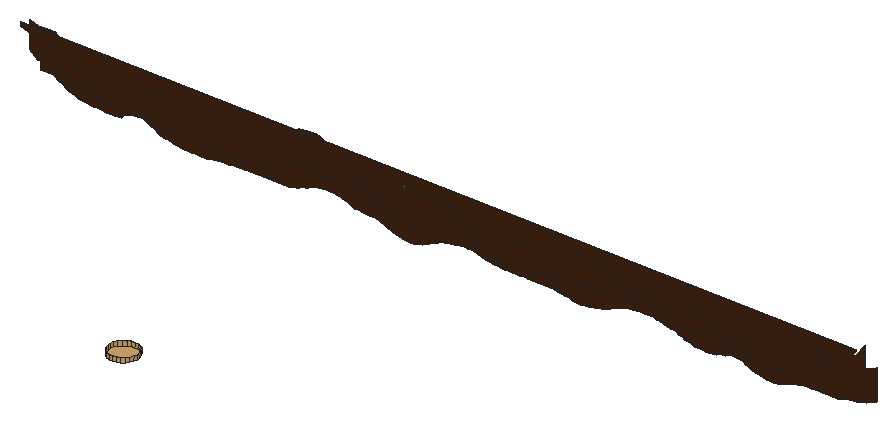
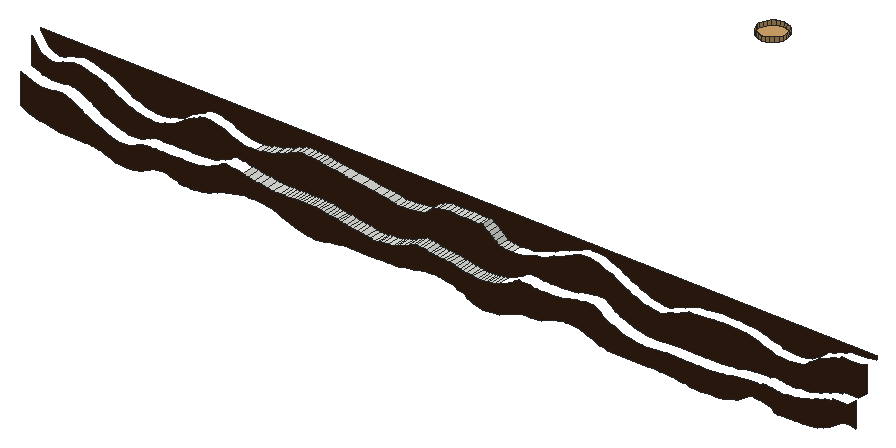
# SketchUp Ruby script. Lengths in inches.
U = 1.inch
M = Sketchup.active_model
def pt(a) = Geom::Point3d.new(a.map { |v| v * U })
def face(e, loops, mat)
  f = e.add_face(loops[0].map { |a| pt(a) })
  loops[1..].each { |l| e.add_face(l.map { |a| pt(a) }).erase! }
  f.material = f.back_material = mat if mat
  f
end
# faces: each face lists its corners as indices into pts; further lists are holes
def faces(e, pts, list, mat = nil) = list.each { |f| face(e, (f[0].is_a?(Array) ? f : [f]).map { |l| l.map { |i| pts[i] } }, mat) }
# xy, xz, yz: faces in a plane at the given z, y or x. An outline is a flat list of corners, or four numbers for a rectangle; further outlines are holes
def ring(l) = l.size == 4 ? [[l[0], l[1]], [l[2], l[1]], [l[2], l[3]], [l[0], l[3]]] : l.each_slice(2).to_a
def flat(e, list, mat, &to3) = list.each { |f| face(e, (f[0].is_a?(Array) ? f : [f]).map { |l| ring(l).map { |u, v| to3.(u, v) } }, mat) }
def xy(e, z, list, mat = nil) = flat(e, list, mat) { |x, y| [x, y, z] }
def xz(e, y, list, mat = nil) = flat(e, list, mat) { |x, z| [x, y, z] }
def yz(e, x, list, mat = nil) = flat(e, list, mat) { |y, z| [x, y, z] }
def lines(e, pts, list) = list.each { |a, b| e.add_line(pt(pts[a]), pt(pts[b])) }
# prism: a flat outline (further loops are holes) pulled along v
def prism(e, loops, v, mat = nil)
  f = face(e, loops, mat); d = Geom::Vector3d.new(v.map { |x| x * U })
  f.pushpull(f.normal.samedirection?(d) ? d.length : -d.length)
end
def box(e, o, s, mat = nil) = prism(e, [[o, [o[0] + s[0], o[1], o[2]], [o[0] + s[0], o[1] + s[1], o[2]], [o[0], o[1] + s[1], o[2]]]], [0, 0, s[2]], mat)
def at(x, y, z, deg = 0) = Geom::Transformation.translation(pt([x, y, z])) * Geom::Transformation.rotation(ORIGIN, Z_AXIS, deg.degrees)
def axes(o, x, y, z) = Geom::Transformation.new([*x, 0, *y, 0, *z, 0, *pt(o).to_a, 1])
def part(name) = M.definitions.add(name)
# library, detail: a bought-in or finely detailed component or shape, given as its bounding box
def library(name, o, s) = part(name).tap { |d| box(d.entities, o, s) }
def detail(e, o, s) = box(e.add_group.entities, o, s)
def put(e, d, t, mat = nil) = e.add_instance(d, t).tap { |i| i.material = mat if mat }
def group(e, t, mat = nil) = e.add_group.tap { |g| g.transformation = t; g.material = mat if mat }.entities
root = M.entities
M.materials.add("[Field Square Tile]").color = [211, 167, 108]
M.materials.add("[Wood Veneer 01]").color = [66, 38, 20]
xy(root,243.05,[[2994.54,2398.8,2995.22,2401.37]])
xy(root,243.07,[[2992.6875,2398.8,2993.27,2401.37]])
xy(root,243.09,[[2989.375,2398.8,2989.9,2401.37],[2989.9,2398.8,2990.42,2401.37],[2990.42,2398.8,2991.08,2401.37],[2991.08,2398.8,2991.53,2401.37]])
xy(root,249.21,[[2962.17,2396.68,2963.06,2398.8]])
xy(root,249.22,[[2963.78,2396.68,2964.6875,2398.8]])
xy(root,249.23,[[2965.33,2396.68,2966.23,2398.8]])
xy(root,250.6875,[[2960.72,2328.39,2960.06,2328.48,2959.44,2328.74,2958.91,2329.14,2958.5,2329.68,2958.25,2330.29,2958.16,2330.96,2958.25,2331.62,2958.5,2332.24,2958.91,2332.77,2959.44,2333.18,2960.06,2333.43,2960.72,2333.52,2961.38,2333.43,2962,2333.18,2962.53,2332.77,2962.94,2332.24,2963.2,2331.62,2963.28,2330.96,2963.2,2330.29,2962.94,2329.68,2962.53,2329.14,2962,2328.74,2961.38,2328.48]],"[Field Square Tile]")
xz(root,2396.68,[[3020.59,244.87,3021.5,245.01,3022.4375,245.12,3023.2,245.25,3023.96,245.41,3024.59,245.78,3025.39,245.88,3026.1,246.16,3026.7,246.57,3027.49,246.9,3028.09,247.35,3028.76,247.62,3029.35,248.06,3030.11,248.32,3031.22,248.66,3032,248.79,3032.86,249.19,3033.53,249.32,3034.46,249.41,3035.31,249.48,3036.06,249.21,3036.7,248.96,3037.4,248.9,3038.2,248.42,3038.91,248.3,3039.62,248.22,3040.4375,248.56,3041.37,249.02,3043.1,251.16,3043.1,251.5,2889.09,251.5,2889.09,250.88,2890.68,250.53,2892.3,250.54,2893.76,250.55,2894.29,250.15,2894.9,249.97,2895.7,249.8,2896.37,249.41,2897.04,249.2,2897.81,249.01,2898.3,248.51,2898.93,248.07,2899.58,247.72,2900.22,247.25,2900.77,246.88,2901.49,246.73,2902.15,246.62,2902.89,246.54,2903.67,246.51,2904.45,246.58,2905.25,246.59,2906.05,246.69,2906.76,247.03,2907.45,247.2,2908.42,247.39,2909.05,247.78,2909.83,247.89,2910.83,248.18,2911.47,248.29,2912.36,248.35,2913.09,248.4,2914.08,248.4375,2914.74,248.46,2915.63,248.47,2916.37,248.48,2917.26,248.49,2917.99,248.39,2919.39,248.28,2920.42,248.15,2921.24,248.11,2922.04,248.08,2922.88,247.66,2923.51,247.46,2924.19,247.08,2924.875,246.94,2925.73,246.66,2926.34,246.35,2927.11,246.05,2928.01,246.13,2928.72,246.29,2929.52,246.41,2930.43,246.55,2931.16,246.92,2931.77,247.12,2932.45,247.31,2933.02,247.71,2933.95,248.03,2934.66,248.46,2935.44,248.82,2936.16,249.37,2936.95,249.5625,2937.85,249.9,2938.77,250.35,2939.43,250.49,2940.24,250.6,2941.26,250.58,2941.9,250.61,2942.52,250.32,2943.21,250.0625,2943.87,249.68,2944.63,249.46,2945.52,248.95,2946.74,248.69,2947.65,248.26,2948.25,247.9,2949.38,247.66,2949.96,247.53,2950.64,247.25,2951.45,246.95,2952.14,246.75,2952.93,246.66,2953.64,246.59,2954.53,246.55,2955.46,246.63,2956.2,246.74,2956.93,246.87,2957.54,247.42,2958.21,247.96,2958.78,248.44,2959.52,248.85,2959.99,249.34,2960.72,249.125,2961.49,249.17,2962.17,249.21,2963.06,249.21,2963.78,249.22,2964.6875,249.22,2965.33,249.23,2966.23,249.23,2966.97,249.24,2967.77,249.14,2968.4,248.82,2969.19,248.54,2969.89,248.04,2970.58,247.48,2971.47,247.29,2972.29,247.15,2973.02,247.05,2973.74,247,2974.65,246.96,2975.375,246.94,2976.29,247.04,2977.35,247.36,2978.53,247.43,2980.18,247.6,2982.16,247.98,2984.36,248.1875,2985.97,248.49,2987.22,248.62,2988.16,248.69,2988.84,248.75,2989.5,249.09,2990.2,249.18,2990.98,249.13,2991.68,249.17,2992.38,249.18,2993.28,249.29,2994.01,249.21,2994.62,248.8,2995.3125,248.73,2996.09,248.26,2996.79,248.02,2997.59,247.8125,2998.3,247.4,2999.21,247.27,2999.95,247.18,3000.875,246.91,3001.74,246.84,3002.69,246.79,3003.47,246.75,3004.22,246.83,3005.26,247.25,3006.13,247.55,3006.8,247.66,3007.43,248.16,3008.22,248.41,3008.92,248.52,3009.62,248.72,3010.32,248.8,3011.21,248.85,3012.04,248.6875,3012.58,248.26,3013.27,248.06,3014.16,247.55,3014.87,247.19,3015.68,246.63,3016.3125,246.13,3016.9,245.83,3017.58,245.67,3018.45,245.46,3019.16,245.0625,3019.875,244.95]],"[Wood Veneer 01]")
xz(root,2398.8,[[3024.59,241.09,3025.16,241.14,3025.8,241.35,3026.39,241.46,3027.33,241.85,3028.33,242.23,3028.89,242.42,3029.61,242.61,3030.125,242.91,3030.5,243.14,3031.04,243.52,3031.52,243.71,3031.85,244.02,3032.29,244.21,3032.88,244.57,3033.35,244.76,3033.97,245.125,3034.47,245.32,3034.95,245.41,3035.5,245.48,3035.99,245.59,3036.52,245.55,3037.13,245.35,3037.62,245.31,3038.17,245.27,3038.73,245.24,3039.29,245.22,3039.85,245.34,3040.48,245.42,3041.0625,245.52,3041.44,245.76,3041.91,245.9,3043.1,246.43,3043.1,251.16,3041.37,249.02,3040.4375,248.56,3039.62,248.22,3038.91,248.3,3038.2,248.42,3037.4,248.9,3036.7,248.96,3036.06,249.21,3035.31,249.48,3034.46,249.41,3033.53,249.32,3032.86,249.19,3032,248.79,3031.22,248.66,3030.11,248.32,3029.35,248.06,3028.76,247.62,3028.09,247.35,3027.49,246.9,3026.7,246.57,3026.1,246.16,3025.39,245.88,3024.59,245.78,3023.96,245.41,3023.2,245.25,3022.4375,245.12,3021.5,245.01,3020.59,244.87,3019.875,244.95,3019.16,245.0625,3018.45,245.46,3017.58,245.67,3016.9,245.83,3016.3125,246.13,3015.68,246.63,3014.87,247.19,3014.16,247.55,3013.27,248.06,3012.58,248.26,3012.04,248.6875,3011.21,248.85,3010.32,248.8,3009.62,248.72,3008.92,248.52,3008.22,248.41,3007.43,248.16,3006.8,247.66,3006.13,247.55,3005.26,247.25,3004.22,246.83,3003.47,246.75,3002.69,246.79,3001.74,246.84,3000.875,246.91,2999.95,247.18,2999.21,247.27,2998.3,247.4,2997.59,247.8125,2996.79,248.02,2996.09,248.26,2995.3125,248.73,2994.62,248.8,2994.01,249.21,2993.28,249.29,2992.38,249.18,2991.68,249.17,2990.98,249.13,2990.2,249.18,2989.5,249.09,2988.84,248.75,2988.16,248.69,2987.22,248.62,2985.97,248.49,2984.36,248.1875,2982.16,247.98,2980.18,247.6,2978.53,247.43,2977.35,247.36,2976.29,247.04,2975.375,246.94,2974.65,246.96,2973.74,247,2973.02,247.05,2972.29,247.15,2971.47,247.29,2970.58,247.48,2969.89,248.04,2969.19,248.54,2968.4,248.82,2967.77,249.14,2966.97,249.24,2966.23,249.23,2965.33,249.23,2964.6875,249.22,2963.78,249.22,2963.06,249.21,2962.17,249.21,2961.49,249.17,2960.72,249.125,2959.99,249.34,2959.52,248.85,2958.78,248.44,2958.21,247.96,2957.54,247.42,2956.93,246.87,2956.2,246.74,2955.46,246.63,2954.53,246.55,2953.64,246.59,2952.93,246.66,2952.14,246.75,2951.45,246.95,2950.64,247.25,2949.96,247.53,2949.38,247.66,2948.25,247.9,2947.65,248.26,2946.74,248.69,2945.52,248.95,2944.63,249.46,2943.87,249.68,2943.21,250.0625,2942.52,250.32,2941.9,250.61,2941.26,250.58,2940.24,250.6,2939.43,250.49,2938.77,250.35,2937.85,249.9,2936.95,249.5625,2936.16,249.37,2935.44,248.82,2934.66,248.46,2933.95,248.03,2933.02,247.71,2932.45,247.31,2931.77,247.12,2931.16,246.92,2930.43,246.55,2929.52,246.41,2928.72,246.29,2928.01,246.13,2927.11,246.05,2926.34,246.35,2925.73,246.66,2924.875,246.94,2924.19,247.08,2923.51,247.46,2922.88,247.66,2922.04,248.08,2921.24,248.11,2920.42,248.15,2919.39,248.28,2917.99,248.39,2917.26,248.49,2916.37,248.48,2915.63,248.47,2914.74,248.46,2914.08,248.4375,2913.09,248.4,2912.36,248.35,2911.47,248.29,2910.83,248.18,2909.83,247.89,2909.05,247.78,2908.42,247.39,2907.45,247.2,2906.76,247.03,2906.05,246.69,2905.25,246.59,2904.45,246.58,2903.67,246.51,2902.89,246.54,2902.15,246.62,2901.49,246.73,2900.77,246.88,2900.22,247.25,2899.58,247.72,2898.93,248.07,2898.3,248.51,2897.81,249.01,2897.04,249.2,2896.37,249.41,2895.7,249.8,2894.9,249.97,2894.29,250.15,2893.76,250.55,2892.3,250.54,2890.68,250.53,2889.09,250.88,2889.09,246.2,2890.66,244.96,2892.05,244.9375,2893.3,244.92,2893.52,244.61,2894.08,244.54,2894.84,244.41,2895.51,244.11,2896.03,243.95,2896.69,243.79,2897.21,243.48,2897.85,243.3,2898.4375,243.14,2898.92,243.06,2899.64,242.85,2900.22,242.78,2901.03,242.73,2901.57,242.68,2902.24,242.51,2902.76,242.46,2903.3,242.58,2903.93,242.57,2904.56,242.81,2905.13,242.86,2905.69,242.89,2906.33,242.92,2906.76,242.625,2907.37,242.65,2907.92,242.62,2908.55,242.58,2909.11,242.57,2909.75,242.48,2910.41,242.38,2911.07,242.34,2911.74,242.24,2912.91,241.96,2913.68,241.89,2914.5,241.83,2915.1,241.78,2915.87,241.75,2916.32,241.74,2916.87,241.72,2918.13,241.7,2918.86,241.69,2919.53,241.68,2920.12,241.68,2920.61,241.67,2921.3125,241.74,2921.88,241.75,2923.88,241.75,2924.37,241.67,2924.9,241.66,2925.51,241.57,2926.05,241.53,2926.67,241.51,2927.22,241.49,2927.92,241.48,2928.58,241.47,2929.15,241.46,2929.86,241.6,2930.59,241.85,2931.26,241.91,2932.16,242.1,2932.93,242.46,2933.63,242.78,2934.4,242.97,2934.93,243.23,2935.33,243.48,2935.85,243.72,2936.1875,244.12,2936.66,244.39,2937.14,244.73,2937.625,244.87,2938.21,244.95,2938.89,245.01,2939.54,244.81,2940.11,244.7,2940.59,244.67,2941.2,244.55,2941.74,244.51,2942.2,244.25,2942.95,244.11,2943.51,244.04,2944.13,243.99,2944.85,243.95,2945.35,243.93,2946.04,243.91,2946.61,243.89,2947.31,243.88,2947.96,243.94,2948.6,243.95,2949.16,244.1,2949.79,244.13,2950.27,244.15,2950.79,244.17,2951.31,244.18,2951.91,243.8,2952.45,243.43,2953.06,243.09,2953.45,242.875,2953.95,242.68,2954.54,242.51,2955.05,242.21,2955.65,242.11,2956.33,241.96,2956.89,241.89,2957.35,241.85,2957.87,241.8125,2958.38,241.79,2958.96,241.78,2959.63,241.91,2960.1,241.93,2960.77,242.09,2961.54,242.2,2962.04,242.24,2962.65,242.42,2963.2,242.47,2963.95,242.71,2964.59,242.78,2965.07,242.82,2965.76,242.85,2966.46,242.87,2967.01,243.02,2967.63,243.05,2968.18,243.29,2968.86,243.35,2969.41,243.39,2970.01,243.42,2970.78,243.14,2971.35,242.9375,2971.9,242.65,2972.52,242.39,2973.28,242.14,2973.92,241.89,2974.41,241.78,2975.46,241.63,2976.23,241.56,2976.83,241.51,2977.28,241.48,2977.8,241.46,2978.67,241.51,2979.39,241.59,2980.33,241.82,2981.11,241.87,2981.875,241.98,2982.49,242.02,2983.14,242.19,2983.84,242.38,2984.33,242.4375,2984.85,242.48,2985.51,242.58,2986.04,242.61,2986.625,242.77,2987.08,242.95,2987.64,243.01,2988.15,243.05,2988.72,243.08,2989.375,243.09,2991.53,243.09,2992.1,243.08,2992.6875,243.07,2993.27,243.07,2993.93,243.0625,2994.54,243.05,2995.22,243.05,2996.49,243.1,2997.66,243.17,2998.8,243.4,3000.0625,243.52,3001.19,243.71,3002.09,243.99,3002.79,244.08,3003.49,244.21,3004.07,244.27,3004.61,244.3,3005.28,244.39,3005.875,244.19,3006.25,243.88,3006.73,243.59,3007.28,243.33,3007.83,243.22,3008.32,242.92,3008.8,242.75,3009.36,242.6,3009.92,242.52,3010.48,242.47,3011.0625,242.43,3011.64,242.4,3012.22,242.39,3012.8,242.37,3013.38,242.36,3013.97,242.35,3015.13,242.33,3015.71,242.33,3016.43,242.32,3016.9,242.3125,3017.54,242.3,3018.21,242.3,3018.66,242.29,3019.3,242.28,3019.8125,242.28,3020.44,242.2,3021.02,241.97,3021.59,241.84,3022.1,241.57,3022.52,241.33,3022.99,241.24,3023.52,241.17,3023.99,241.12]],"[Wood Veneer 01]")
xz(root,2401.37,[[2957.95,236.98,2958.63,237.22,2959.48,237.43,2960.1,237.74,2960.8,238.02,2961.24,238.375,2961.8,238.51,2962.4375,238.76,2963.08,239.12,2963.66,239.22,2964.66,239.31,2965.47,239.54,2965.96,239.6,2966.58,239.65,2967.17,239.69,2967.73,239.7,2968.46,239.72,2969.07,239.56,2969.74,239.44,2970.59,239.16,2971.14,239.07,2971.91,238.93,2972.79,238.78,2973.27,238.73,2973.94,238.6875,2974.63,238.66,2975.3,238.65,2976.08,238.64,2976.7,238.63,2977.39,238.625,2978.25,238.625,2978.81,238.62,2983.7,238.62,2984.39,238.45,2985.15,238.25,2985.77,238.19,2986.54,238.15,2987.17,237.86,2987.94,237.79,2988.65,237.74,2989.52,237.87,2990.17,237.88,2991.29,238.14,2992.51,238.46,2993.26,238.72,2994.14,239.08,2994.93,239.375,2995.67,239.75,2996.32,239.97,2996.94,240.17,2997.62,240.27,2998.3,240.33,2998.99,240.37,2999.68,240.4,3000.375,240.41,3000.9,240.42,3001.48,240.43,3002.05,240.43,3002.7,240.27,3003.28,240.23,3003.93,239.96,3004.6875,239.8,3005.3,239.65,3006.0625,239.5,3006.6875,239.18,3007.37,239.01,3007.89,238.67,3008.46,238.56,3009.12,238.48,3009.6875,238.26,3010.26,238.19,3011.08,238.15,3011.61,238.11,3012.28,238.18,3012.96,238.18,3013.64,238.27,3014.16,238.55,3014.82,238.61,3015.41,238.66,3015.98,239.04,3016.72,239.125,3017.4,239.02,3018.09,238.96,3018.61,238.86,3019.11,238.57,3019.66,238.33,3020.37,238,3021.2,237.71,3021.74,237.59,3022.34,237.51,3022.93,237.45,3023.5,237.42,3024.23,237.4,3024.91,237.47,3025.51,237.5625,3026.2,237.84,3026.88,238.08,3027.57,238.33,3028.1,238.51,3028.67,238.6,3029.33,238.74,3029.91,238.8,3030.48,238.83,3031.22,238.86,3031.98,238.875,3032.52,238.88,3033.2,238.89,3033.88,238.89,3034.64,238.9,3036.03,238.9,3036.66,239.15,3037.43,239.28,3038.23,239.42,3038.95,239.49,3039.5,239.53,3040.1875,239.81,3040.71,239.96,3041.27,240.1,3043.1,240.89,3043.1,246.43,3041.91,245.9,3041.44,245.76,3041.0625,245.52,3040.48,245.42,3039.85,245.34,3039.29,245.22,3038.73,245.24,3038.17,245.27,3037.62,245.31,3037.13,245.35,3036.52,245.55,3035.99,245.59,3035.5,245.48,3034.95,245.41,3034.47,245.32,3033.97,245.125,3033.35,244.76,3032.88,244.57,3032.29,244.21,3031.85,244.02,3031.52,243.71,3031.04,243.52,3030.5,243.14,3030.125,242.91,3029.61,242.61,3028.89,242.42,3028.33,242.23,3027.33,241.85,3026.39,241.46,3025.8,241.35,3025.16,241.14,3024.59,241.09,3023.99,241.12,3023.52,241.17,3022.99,241.24,3022.52,241.33,3022.1,241.57,3021.59,241.84,3021.02,241.97,3020.44,242.2,3019.8125,242.28,3019.3,242.28,3018.66,242.29,3018.21,242.3,3017.54,242.3,3016.9,242.3125,3016.43,242.32,3015.71,242.33,3015.13,242.33,3013.97,242.35,3013.38,242.36,3012.8,242.37,3012.22,242.39,3011.64,242.4,3011.0625,242.43,3010.48,242.47,3009.92,242.52,3009.36,242.6,3008.8,242.75,3008.32,242.92,3007.83,243.22,3007.28,243.33,3006.73,243.59,3006.25,243.88,3005.875,244.19,3005.28,244.39,3004.61,244.3,3004.07,244.27,3003.49,244.21,3002.79,244.08,3002.09,243.99,3001.19,243.71,3000.0625,243.52,2998.8,243.4,2997.66,243.17,2996.49,243.1,2995.22,243.05,2994.54,243.05,2993.93,243.0625,2993.27,243.07,2992.6875,243.07,2992.1,243.08,2991.53,243.09,2989.375,243.09,2988.72,243.08,2988.15,243.05,2987.64,243.01,2987.08,242.95,2986.625,242.77,2986.04,242.61,2985.51,242.58,2984.85,242.48,2984.33,242.4375,2983.84,242.38,2983.14,242.19,2982.49,242.02,2981.875,241.98,2981.11,241.87,2980.33,241.82,2979.39,241.59,2978.67,241.51,2977.8,241.46,2977.28,241.48,2976.83,241.51,2976.23,241.56,2975.46,241.63,2974.41,241.78,2973.92,241.89,2973.28,242.14,2972.52,242.39,2971.9,242.65,2971.35,242.9375,2970.78,243.14,2970.01,243.42,2969.41,243.39,2968.86,243.35,2968.18,243.29,2967.63,243.05,2967.01,243.02,2966.46,242.87,2965.76,242.85,2965.07,242.82,2964.59,242.78,2963.95,242.71,2963.2,242.47,2962.65,242.42,2962.04,242.24,2961.54,242.2,2960.77,242.09,2960.1,241.93,2959.63,241.91,2958.96,241.78,2958.38,241.79,2957.87,241.8125,2957.35,241.85,2956.89,241.89,2956.33,241.96,2955.65,242.11,2955.05,242.21,2954.54,242.51,2953.95,242.68,2953.45,242.875,2953.06,243.09,2952.45,243.43,2951.91,243.8,2951.31,244.18,2950.79,244.17,2950.27,244.15,2949.79,244.13,2949.16,244.1,2948.6,243.95,2947.96,243.94,2947.31,243.88,2946.61,243.89,2946.04,243.91,2945.35,243.93,2944.85,243.95,2944.13,243.99,2943.51,244.04,2942.95,244.11,2942.2,244.25,2941.74,244.51,2941.2,244.55,2940.59,244.67,2940.11,244.7,2939.54,244.81,2938.89,245.01,2938.21,244.95,2937.625,244.87,2937.14,244.73,2936.66,244.39,2936.1875,244.12,2935.85,243.72,2935.33,243.48,2934.93,243.23,2934.4,242.97,2933.63,242.78,2932.93,242.46,2932.16,242.1,2931.26,241.91,2930.59,241.85,2929.86,241.6,2929.15,241.46,2928.58,241.47,2927.92,241.48,2927.22,241.49,2926.67,241.51,2926.05,241.53,2925.51,241.57,2924.9,241.66,2924.37,241.67,2923.88,241.75,2921.88,241.75,2921.3125,241.74,2920.61,241.67,2920.12,241.68,2919.53,241.68,2918.86,241.69,2918.13,241.7,2916.87,241.72,2916.32,241.74,2915.87,241.75,2915.1,241.78,2914.5,241.83,2913.68,241.89,2912.91,241.96,2911.74,242.24,2911.07,242.34,2910.41,242.38,2909.75,242.48,2909.11,242.57,2908.55,242.58,2907.92,242.62,2907.37,242.65,2906.76,242.625,2906.33,242.92,2905.69,242.89,2905.13,242.86,2904.56,242.81,2903.93,242.57,2903.3,242.58,2902.76,242.46,2902.24,242.51,2901.57,242.68,2901.03,242.73,2900.22,242.78,2899.64,242.85,2898.92,243.06,2898.4375,243.14,2897.85,243.3,2897.21,243.48,2896.69,243.79,2896.03,243.95,2895.51,244.11,2894.84,244.41,2894.08,244.54,2893.52,244.61,2893.3,244.92,2892.05,244.9375,2890.66,244.96,2889.09,246.2,2889.09,241.52,2890.3,241.69,2891.57,241.55,2892.59,240.85,2893.13,240.59,2893.73,240.2,2894.52,239.86,2894.97,239.64,2895.53,239.52,2896.04,239.19,2896.82,239.09,2897.51,239.03,2898.19,238.97,2898.89,238.94,2899.59,238.93,2900.28,238.92,2901.32,238.82,2901.83,238.8,2902.7,238.79,2903.44,238.77,2903.97,238.9375,2904.53,239.55,2905.11,239.69,2905.66,239.88,2906.39,239.99,2906.98,240.05,2907.64,240.09,2908.33,240.11,2909.03,239.71,2909.49,239.38,2910.07,239.11,2910.65,238.74,2911.3,238.43,2912.21,238.31,2912.68,238.21,2913.62,237.9,2914.28,237.82,2914.97,237.76,2915.68,237.71,2916.29,237.68,2916.89,237.67,2917.64,237.66,2918.33,237.65,2919.64,237.65,2920.31,237.89,2921.07,237.94,2921.6875,237.98,2922.54,238.1,2923.09,238.13,2923.85,238.15,2924.48,238.26,2925.23,238.28,2925.86,238.3,2926.71,238.32,2927.43,238.33,2928.66,238.33,2929.34,238.34,2934.91,238.34,2935.42,238.59,2936.24,238.72,2936.93,238.86,2937.44,239.18,2938.03,239.35,2938.59,239.52,2939.14,239.85,2939.78,240.03,2940.4375,240.12,2941.11,240.19,2941.875,240.23,2942.58,240.25,2943.2,240.27,2943.98,240.11,2944.61,239.92,2945.3,239.7,2945.83,239.53,2946.41,239.29,2947.07,239.04,2947.65,238.94,2948.22,238.875,2948.97,238.83,2949.73,238.8,2950.27,238.79,2950.94,238.78,2951.72,238.43,2952.5,238.28,2953.0625,237.96,2954,237.68,2954.67,237.33,2955.2,237.2,2955.89,237.11,2956.65,237.04,2957.34,237.01]],"[Wood Veneer 01]")
p = [[2976.23,2398.8,241.56],[2976.23,2401.37,241.56],[2976.83,2401.37,241.51],[2976.83,2398.8,241.51],[2977.28,2401.37,241.48],[2977.28,2398.8,241.48],
  [2977.8,2401.37,241.46],[2977.8,2398.8,241.46],[2978.67,2401.37,241.51],[2978.67,2398.8,241.51],[2979.39,2401.37,241.59],[2979.39,2398.8,241.59],
  [2974.41,2398.8,241.78],[2974.41,2401.37,241.78],[2975.46,2401.37,241.63],[2975.46,2398.8,241.63],[2980.33,2401.37,241.82],[2980.33,2398.8,241.82],
  [2956.89,2398.8,241.89],[2956.89,2401.37,241.89],[2957.35,2401.37,241.85],[2957.35,2398.8,241.85],[2957.87,2401.37,241.8125],[2957.87,2398.8,241.8125],
  [2958.38,2401.37,241.79],[2958.38,2398.8,241.79],[2958.96,2401.37,241.78],[2958.96,2398.8,241.78],[2959.63,2401.37,241.91],[2959.63,2398.8,241.91],
  [2973.92,2398.8,241.89],[2973.92,2401.37,241.89],[2981.11,2401.37,241.87],[2981.11,2398.8,241.87],[2956.33,2398.8,241.96],[2956.33,2401.37,241.96],
  [2960.1,2401.37,241.93],[2960.1,2398.8,241.93],[2960.77,2401.37,242.09],[2960.77,2398.8,242.09],[2973.28,2398.8,242.14],[2973.28,2401.37,242.14],
  [2981.875,2401.37,241.98],[2981.875,2398.8,241.98],[2955.65,2398.8,242.11],[2955.65,2401.37,242.11],[2982.49,2401.37,242.02],[2982.49,2398.8,242.02],
  [2983.14,2401.37,242.19],[2983.14,2398.8,242.19],[2955.05,2398.8,242.21],[2955.05,2401.37,242.21],[2961.54,2401.37,242.2],[2961.54,2398.8,242.2],
  [2972.52,2398.8,242.39],[2972.52,2401.37,242.39],[2962.04,2401.37,242.24],[2962.04,2398.8,242.24],[2962.65,2401.37,242.42],[2962.65,2398.8,242.42],
  [2983.84,2401.37,242.38],[2983.84,2398.8,242.38],[2963.2,2401.37,242.47],[2963.2,2398.8,242.47],[2971.9,2398.8,242.65],[2971.9,2401.37,242.65],
  [2984.33,2401.37,242.4375],[2984.33,2398.8,242.4375],[2984.85,2401.37,242.48],[2984.85,2398.8,242.48],[2963.95,2401.37,242.71],[2963.95,2398.8,242.71],
  [2985.51,2401.37,242.58],[2985.51,2398.8,242.58],[2971.35,2398.8,242.9375],[2971.35,2401.37,242.9375],[2986.04,2401.37,242.61],[2986.04,2398.8,242.61],
  [2986.625,2401.37,242.77],[2986.625,2398.8,242.77],[2964.59,2401.37,242.78],[2964.59,2398.8,242.78],[2965.07,2401.37,242.82],[2965.07,2398.8,242.82],
  [2965.76,2401.37,242.85],[2965.76,2398.8,242.85],[2987.08,2401.37,242.95],[2987.08,2398.8,242.95],[2966.46,2401.37,242.87],[2966.46,2398.8,242.87],
  [2967.01,2401.37,243.02],[2967.01,2398.8,243.02],[2970.78,2398.8,243.14],[2970.78,2401.37,243.14],[2967.63,2401.37,243.05],[2967.63,2398.8,243.05],
  [2987.64,2401.37,243.01],[2987.64,2398.8,243.01],[2988.15,2401.37,243.05],[2988.15,2398.8,243.05],[2988.72,2401.37,243.08],[2988.72,2398.8,243.08],
  [2995.22,2398.8,243.05],[2995.22,2401.37,243.05],[2996.49,2401.37,243.1],[2996.49,2398.8,243.1],[2968.18,2401.37,243.29],[2968.18,2398.8,243.29],
  [2970.01,2398.8,243.42],[2970.01,2401.37,243.42],[2989.375,2401.37,243.09],[2989.375,2398.8,243.09],[2991.53,2398.8,243.09],[2991.53,2401.37,243.09],
  [2992.1,2401.37,243.08],[2992.1,2398.8,243.08],[2992.6875,2401.37,243.07],[2992.6875,2398.8,243.07],[2993.27,2398.8,243.07],[2993.27,2401.37,243.07],
  [2993.93,2401.37,243.0625],[2993.93,2398.8,243.0625],[2994.54,2401.37,243.05],[2994.54,2398.8,243.05],[2997.66,2401.37,243.17],[2997.66,2398.8,243.17],
  [2998.8,2401.37,243.4],[2998.8,2398.8,243.4],[2968.86,2401.37,243.35],[2968.86,2398.8,243.35],[2969.41,2401.37,243.39],[2969.41,2398.8,243.39],
  [3000.0625,2401.37,243.52],[3000.0625,2398.8,243.52],[3001.19,2401.37,243.71],[3001.19,2398.8,243.71],[3002.09,2401.37,243.99],[3002.09,2398.8,243.99],
  [2954.53,2396.68,246.55],[2954.53,2398.8,246.55],[2955.46,2398.8,246.63],[2955.46,2396.68,246.63],[2956.2,2398.8,246.74],[2956.2,2396.68,246.74],
  [2956.93,2398.8,246.87],[2956.93,2396.68,246.87],[3000.875,2396.68,246.91],[3000.875,2398.8,246.91],[3001.74,2398.8,246.84],[3001.74,2396.68,246.84],
  [2957.54,2398.8,247.42],[2957.54,2396.68,247.42],[2974.65,2396.68,246.96],[2974.65,2398.8,246.96],[2975.375,2398.8,246.94],[2975.375,2396.68,246.94],
  [2976.29,2398.8,247.04],[2976.29,2396.68,247.04],[2999.95,2396.68,247.18],[2999.95,2398.8,247.18],[2972.29,2396.68,247.15],[2972.29,2398.8,247.15],
  [2973.02,2398.8,247.05],[2973.02,2396.68,247.05],[2973.74,2398.8,247],[2973.74,2396.68,247],[2977.35,2398.8,247.36],[2977.35,2396.68,247.36],
  [2971.47,2396.68,247.29],[2971.47,2398.8,247.29],[2999.21,2396.68,247.27],[2999.21,2398.8,247.27],[2970.58,2396.68,247.48],[2970.58,2398.8,247.48],
  [2998.3,2396.68,247.4],[2998.3,2398.8,247.4],[2958.21,2398.8,247.96],[2958.21,2396.68,247.96],[2978.53,2398.8,247.43],[2978.53,2396.68,247.43],
  [2980.18,2398.8,247.6],[2980.18,2396.68,247.6],[2997.59,2396.68,247.8125],[2997.59,2398.8,247.8125],[2969.89,2396.68,248.04],[2969.89,2398.8,248.04],
  [2982.16,2398.8,247.98],[2982.16,2396.68,247.98],[2996.79,2396.68,248.02],[2996.79,2398.8,248.02],[2958.78,2398.8,248.44],[2958.78,2396.68,248.44],
  [2969.19,2396.68,248.54],[2969.19,2398.8,248.54],[2984.36,2398.8,248.1875],[2984.36,2396.68,248.1875],[2996.09,2396.68,248.26],[2996.09,2398.8,248.26],
  [2985.97,2398.8,248.49],[2985.97,2396.68,248.49],[2995.3125,2396.68,248.73],[2995.3125,2398.8,248.73],[2959.52,2398.8,248.85],[2959.52,2396.68,248.85],
  [2968.4,2396.68,248.82],[2968.4,2398.8,248.82],[2987.22,2398.8,248.62],[2987.22,2396.68,248.62],[2988.16,2398.8,248.69],[2988.16,2396.68,248.69],
  [2988.84,2398.8,248.75],[2988.84,2396.68,248.75],[2994.62,2396.68,248.8],[2994.62,2398.8,248.8],[2967.77,2396.68,249.14],[2967.77,2398.8,249.14],
  [2989.5,2398.8,249.09],[2989.5,2396.68,249.09],[2994.01,2396.68,249.21],[2994.01,2398.8,249.21],[2959.99,2398.8,249.34],[2959.99,2396.68,249.34],
  [2960.72,2398.8,249.125],[2960.72,2396.68,249.125],[2961.49,2398.8,249.17],[2961.49,2396.68,249.17],[2966.97,2396.68,249.24],[2966.97,2398.8,249.24],
  [2990.2,2398.8,249.18],[2990.2,2396.68,249.18],[2990.98,2398.8,249.13],[2990.98,2396.68,249.13],[2991.68,2398.8,249.17],[2991.68,2396.68,249.17],
  [2962.17,2398.8,249.21],[2962.17,2396.68,249.21],[2963.06,2396.68,249.21],[2963.06,2398.8,249.21],[2963.78,2398.8,249.22],[2963.78,2396.68,249.22],
  [2964.6875,2396.68,249.22],[2964.6875,2398.8,249.22],[2965.33,2398.8,249.23],[2965.33,2396.68,249.23],[2966.23,2396.68,249.23],[2966.23,2398.8,249.23],
  [2992.38,2398.8,249.18],[2992.38,2396.68,249.18],[2993.28,2398.8,249.29],[2993.28,2396.68,249.29],[2960.72,2328.39,251.5],[2960.06,2328.48,251.5],
  [2960.06,2328.48,250.6875],[2960.72,2328.39,250.6875],[2961.38,2328.48,251.5],[2961.38,2328.48,250.6875],[2959.44,2328.74,251.5],[2959.44,2328.74,250.6875],
  [2962,2328.74,251.5],[2962,2328.74,250.6875],[2958.91,2329.14,251.5],[2958.91,2329.14,250.6875],[2962.53,2329.14,251.5],[2962.53,2329.14,250.6875],
  [2958.5,2329.68,251.5],[2958.5,2329.68,250.6875],[2962.94,2329.68,251.5],[2962.94,2329.68,250.6875],[2958.25,2330.29,251.5],[2958.25,2330.29,250.6875],
  [2963.2,2330.29,251.5],[2963.2,2330.29,250.6875],[2958.16,2330.96,251.5],[2958.16,2330.96,250.6875],[2963.28,2330.96,251.5],[2963.28,2330.96,250.6875],
  [2958.25,2331.62,251.5],[2958.25,2331.62,250.6875],[2963.2,2331.62,251.5],[2963.2,2331.62,250.6875],[2958.5,2332.24,251.5],[2958.5,2332.24,250.6875],
  [2962.94,2332.24,251.5],[2962.94,2332.24,250.6875],[2958.91,2332.77,251.5],[2958.91,2332.77,250.6875],[2962.53,2332.77,251.5],[2962.53,2332.77,250.6875],
  [2959.44,2333.18,251.5],[2959.44,2333.18,250.6875],[2962,2333.18,251.5],[2962,2333.18,250.6875],[2960.06,2333.43,251.5],[2960.06,2333.43,250.6875],
  [2961.38,2333.43,251.5],[2961.38,2333.43,250.6875],[2960.72,2333.52,251.5],[2960.72,2333.52,250.6875]]
faces(root,p,[[0,1,2,3],[3,2,4,5],[5,4,6,7],[7,6,8,9],[9,8,10,11],[12,13,14,15],[15,14,1,0],[11,10,16,17],
  [18,19,20,21],[21,20,22,23],[23,22,24,25],[25,24,26,27],[27,26,28,29],[30,31,13,12],[17,16,32,33],[34,35,19,18],
  [29,28,36,37],[37,36,38,39],[40,41,31,30],[33,32,42,43],[44,45,35,34],[43,42,46,47],[47,46,48,49],[50,51,45,44],
  [39,38,52,53],[54,55,41,40],[53,52,56,57],[57,56,58,59],[49,48,60,61],[59,58,62,63],[64,65,55,54],[61,60,66,67],
  [67,66,68,69],[63,62,70,71],[69,68,72,73],[74,75,65,64],[73,72,76,77],[77,76,78,79],[71,70,80,81],[81,80,82,83],
  [83,82,84,85],[79,78,86,87],[85,84,88,89],[89,88,90,91],[92,93,75,74],[91,90,94,95],[87,86,96,97],[97,96,98,99],
  [99,98,100,101],[102,103,104,105],[95,94,106,107],[108,109,93,92],[101,100,110,111],[112,113,114,115],[115,114,116,117],[118,119,120,121],
  [121,120,122,123],[105,104,124,125],[125,124,126,127],[107,106,128,129],[129,128,130,131],[131,130,109,108],[127,126,132,133],[133,132,134,135],
  [135,134,136,137],[138,139,140,141],[141,140,142,143],[143,142,144,145],[146,147,148,149],[145,144,150,151],[152,153,154,155],[155,154,156,157],
  [158,159,147,146],[160,161,162,163],[163,162,164,165],[165,164,153,152],[157,156,166,167],[168,169,161,160],[170,171,159,158],[172,173,169,168],
  [174,175,171,170],[151,150,176,177],[167,166,178,179],[179,178,180,181],[182,183,175,174],[184,185,173,172],[181,180,186,187],[188,189,183,182],
  [177,176,190,191],[192,193,185,184],[187,186,194,195],[196,197,189,188],[195,194,198,199],[200,201,197,196],[191,190,202,203],[204,205,193,192],
  [199,198,206,207],[207,206,208,209],[209,208,210,211],[212,213,201,200],[214,215,205,204],[211,210,216,217],[218,219,213,212],[203,202,220,221],
  [221,220,222,223],[223,222,224,225],[226,227,215,214],[217,216,228,229],[229,228,230,231],[231,230,232,233],[225,224,234,235],[236,237,238,239],
  [240,241,242,243],[244,245,227,226],[233,232,246,247],[247,246,248,249],[249,248,219,218]])
faces(root,p,[[250,251,252,253],[254,250,253,255],[251,256,257,252],[258,254,255,259],[256,260,261,257],[262,258,259,263],[260,264,265,261],[266,262,263,267],
  [264,268,269,265],[270,266,267,271],[268,272,273,269],[274,270,271,275],[272,276,277,273],[278,274,275,279],[276,280,281,277],[282,278,279,283],
  [280,284,285,281],[286,282,283,287],[284,288,289,285],[290,286,287,291],[288,292,293,289],[294,290,291,295],[292,296,297,293],[296,294,295,297]],"[Field Square Tile]")
